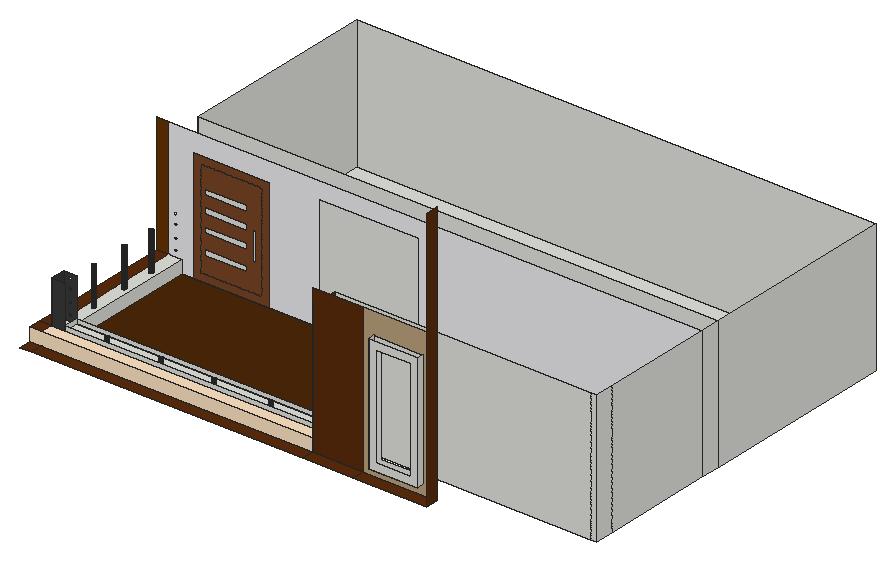
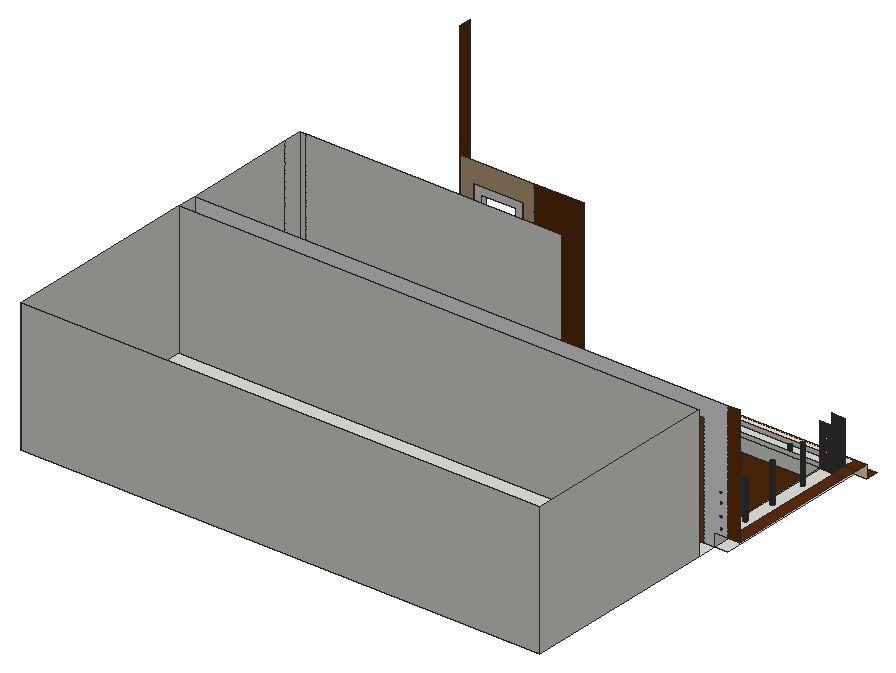
# SketchUp Ruby script. Lengths in inches.
U = 1.inch
M = Sketchup.active_model
def pt(a) = Geom::Point3d.new(a.map { |v| v * U })
def face(e, loops, mat)
  f = e.add_face(loops[0].map { |a| pt(a) })
  loops[1..].each { |l| e.add_face(l.map { |a| pt(a) }).erase! }
  f.material = f.back_material = mat if mat
  f
end
# faces: each face lists its corners as indices into pts; further lists are holes
def faces(e, pts, list, mat = nil) = list.each { |f| face(e, (f[0].is_a?(Array) ? f : [f]).map { |l| l.map { |i| pts[i] } }, mat) }
# xy, xz, yz: faces in a plane at the given z, y or x. An outline is a flat list of corners, or four numbers for a rectangle; further outlines are holes
def ring(l) = l.size == 4 ? [[l[0], l[1]], [l[2], l[1]], [l[2], l[3]], [l[0], l[3]]] : l.each_slice(2).to_a
def flat(e, list, mat, &to3) = list.each { |f| face(e, (f[0].is_a?(Array) ? f : [f]).map { |l| ring(l).map { |u, v| to3.(u, v) } }, mat) }
def xy(e, z, list, mat = nil) = flat(e, list, mat) { |x, y| [x, y, z] }
def xz(e, y, list, mat = nil) = flat(e, list, mat) { |x, z| [x, y, z] }
def yz(e, x, list, mat = nil) = flat(e, list, mat) { |y, z| [x, y, z] }
def lines(e, pts, list) = list.each { |a, b| e.add_line(pt(pts[a]), pt(pts[b])) }
# prism: a flat outline (further loops are holes) pulled along v
def prism(e, loops, v, mat = nil)
  f = face(e, loops, mat); d = Geom::Vector3d.new(v.map { |x| x * U })
  f.pushpull(f.normal.samedirection?(d) ? d.length : -d.length)
end
def box(e, o, s, mat = nil) = prism(e, [[o, [o[0] + s[0], o[1], o[2]], [o[0] + s[0], o[1] + s[1], o[2]], [o[0], o[1] + s[1], o[2]]]], [0, 0, s[2]], mat)
def at(x, y, z, deg = 0) = Geom::Transformation.translation(pt([x, y, z])) * Geom::Transformation.rotation(ORIGIN, Z_AXIS, deg.degrees)
def axes(o, x, y, z) = Geom::Transformation.new([*x, 0, *y, 0, *z, 0, *pt(o).to_a, 1])
def part(name) = M.definitions.add(name)
# library, detail: a bought-in or finely detailed component or shape, given as its bounding box
def library(name, o, s) = part(name).tap { |d| box(d.entities, o, s) }
def detail(e, o, s) = box(e.add_group.entities, o, s)
def put(e, d, t, mat = nil) = e.add_instance(d, t).tap { |i| i.material = mat if mat }
def group(e, t, mat = nil) = e.add_group.tap { |g| g.transformation = t; g.material = mat if mat }.entities
root = M.entities
M.materials.add("[0012_Bisque]").color = [255, 228, 196]
M.materials.add("[0035_Tan]").color = [188, 161, 125]
M.materials.add("[0043_SaddleBrown]").color = [91, 44, 12]
M.materials.add("[Blinds Vertical Pattern]").color = [237, 237, 239]
M.materials.add("[Color C08]").color = [102, 51, 0]
M.materials.add("[Color M07]").color = [58, 58, 58]
M.materials.add("[Leather Red Brown]").color = [76, 40, 8]
M.materials.add("[Wood Veneer 01]").color = [120, 70, 37]
xy(root,141.625,[[73.92,393.34,73.92,538.2,85.98,538.2,85.98,418.04,320.99,418.04,320.99,393.34],[85.98,538.2,560.26,556.28],[85.98,556.28,560.26,737.09]])
xy(root,141.625,[[63.07,382.09,73.92,393.34],[73.92,382.09,320.99,393.34],[320.99,382.09,366.56,393.34],[366.56,382.09,434.25,393.34]],"[0043_SaddleBrown]")
xy(root,141.625,[[85.98,418.04,560.26,538.2]],"[Leather Red Brown]")
xy(root,150.96,[[376.94,386.84,421.82,393.34]])
xy(root,153.1875,[[73.92,404.47,85.98,418.04],[[85.98,404.47,320.99,418.04],[216.94,409.26,217.34,409.31,217.71,409.45,218.03,409.67,218.28,409.95,218.43,410.28,218.48,410.64,218.43,410.99,218.28,411.33,218.03,411.61,217.71,411.83,217.34,411.97,216.94,412.01,216.54,411.97,216.17,411.83,215.85,411.61,215.61,411.33,215.46,410.99,215.4,410.64,215.46,410.28,215.61,409.95,215.85,409.67,216.17,409.45,216.54,409.31],[268.74,409.26,269.14,409.31,269.51,409.45,269.83,409.67,270.08,409.95,270.23,410.28,270.28,410.64,270.23,410.99,270.08,411.33,269.83,411.61,269.51,411.83,269.14,411.97,268.74,412.01,268.34,411.97,267.97,411.83,267.65,411.61,267.41,411.33,267.26,410.99,267.2,410.64,267.26,410.28,267.41,409.95,267.65,409.67,267.97,409.45,268.34,409.31],[168.5,409.26,168.9,409.31,169.27,409.45,169.59,409.67,169.84,409.95,169.99,410.28,170.04,410.64,169.99,410.99,169.84,411.33,169.59,411.61,169.27,411.83,168.9,411.97,168.5,412.01,168.1,411.97,167.73,411.83,167.41,411.61,167.17,411.33,167.02,410.99,166.96,410.64,167.02,410.28,167.17,409.95,167.41,409.67,167.73,409.45,168.1,409.31],[119.01,409.26,119.41,409.31,119.78,409.45,120.1,409.67,120.35,409.95,120.5,410.28,120.55,410.64,120.5,410.99,120.35,411.33,120.1,411.61,119.78,411.83,119.41,411.97,119.01,412.01,118.61,411.97,118.24,411.83,117.92,411.61,117.68,411.33,117.53,410.99,117.47,410.64,117.53,410.28,117.68,409.95,117.92,409.67,118.24,409.45,118.61,409.31]],[119.01,409.26,118.61,409.31,118.24,409.45,117.92,409.67,117.68,409.95,117.53,410.28,117.47,410.64,117.53,410.99,117.68,411.33,117.92,411.61,118.24,411.83,118.61,411.97,119.01,412.01,119.41,411.97,119.78,411.83,120.1,411.61,120.35,411.33,120.5,410.99,120.55,410.64,120.5,410.28,120.35,409.95,120.1,409.67,119.78,409.45,119.41,409.31],[168.5,409.26,168.1,409.31,167.73,409.45,167.41,409.67,167.17,409.95,167.02,410.28,166.96,410.64,167.02,410.99,167.17,411.33,167.41,411.61,167.73,411.83,168.1,411.97,168.5,412.01,168.9,411.97,169.27,411.83,169.59,411.61,169.84,411.33,169.99,410.99,170.04,410.64,169.99,410.28,169.84,409.95,169.59,409.67,169.27,409.45,168.9,409.31],[216.94,409.26,216.54,409.31,216.17,409.45,215.85,409.67,215.61,409.95,215.46,410.28,215.4,410.64,215.46,410.99,215.61,411.33,215.85,411.61,216.17,411.83,216.54,411.97,216.94,412.01,217.34,411.97,217.71,411.83,218.03,411.61,218.28,411.33,218.43,410.99,218.48,410.64,218.43,410.28,218.28,409.95,218.03,409.67,217.71,409.45,217.34,409.31],
  [268.74,409.26,268.34,409.31,267.97,409.45,267.65,409.67,267.41,409.95,267.26,410.28,267.2,410.64,267.26,410.99,267.41,411.33,267.65,411.61,267.97,411.83,268.34,411.97,268.74,412.01,269.14,411.97,269.51,411.83,269.83,411.61,270.08,411.33,270.23,410.99,270.28,410.64,270.23,410.28,270.08,409.95,269.83,409.67,269.51,409.45,269.14,409.31],[[73.92,418.04,85.98,538.2],[80.02,443.08,79.56,443.13,79.14,443.29,78.78,443.54,78.5,443.86,78.33,444.24,78.27,444.64,78.33,445.05,78.5,445.42,78.78,445.75,79.14,445.99,79.56,446.15,80.02,446.2,80.47,446.15,80.89,445.99,81.25,445.75,81.53,445.42,81.71,445.05,81.77,444.64,81.71,444.24,81.53,443.86,81.25,443.54,80.89,443.29,80.47,443.13],[80.02,477.83,79.56,477.88,79.14,478.04,78.78,478.29,78.5,478.61,78.33,478.99,78.27,479.39,78.33,479.8,78.5,480.17,78.78,480.5,79.14,480.74,79.56,480.9,80.02,480.95,80.47,480.9,80.89,480.74,81.25,480.5,81.53,480.17,81.71,479.8,81.77,479.39,81.71,478.99,81.53,478.61,81.25,478.29,80.89,478.04,80.47,477.88],[80.02,508.58,79.56,508.63,79.14,508.79,78.78,509.04,78.5,509.36,78.33,509.74,78.27,510.14,78.33,510.55,78.5,510.92,78.78,511.25,79.14,511.49,79.56,511.65,80.02,511.7,80.47,511.65,80.89,511.49,81.25,511.25,81.53,510.92,81.71,510.55,81.77,510.14,81.71,509.74,81.53,509.36,81.25,509.04,80.89,508.79,80.47,508.63]],[80.02,443.08,79.56,443.13,79.14,443.29,78.78,443.54,78.5,443.86,78.33,444.24,78.27,444.64,78.33,445.05,78.5,445.42,78.78,445.75,79.14,445.99,79.56,446.15,80.02,446.2,80.47,446.15,80.89,445.99,81.25,445.75,81.53,445.42,81.71,445.05,81.77,444.64,81.71,444.24,81.53,443.86,81.25,443.54,80.89,443.29,80.47,443.13],[80.02,477.83,79.56,477.88,79.14,478.04,78.78,478.29,78.5,478.61,78.33,478.99,78.27,479.39,78.33,479.8,78.5,480.17,78.78,480.5,79.14,480.74,79.56,480.9,80.02,480.95,80.47,480.9,80.89,480.74,81.25,480.5,81.53,480.17,81.71,479.8,81.77,479.39,81.71,478.99,81.53,478.61,81.25,478.29,80.89,478.04,80.47,477.88],[80.02,508.58,79.56,508.63,79.14,508.79,78.78,509.04,78.5,509.36,78.33,509.74,78.27,510.14,78.33,510.55,78.5,510.92,78.78,511.25,79.14,511.49,79.56,511.65,80.02,511.7,80.47,511.65,80.89,511.49,81.25,511.25,81.53,510.92,81.71,510.55,81.77,510.14,81.71,509.74,81.53,509.36,81.25,509.04,80.89,508.79,80.47,508.63]])
xy(root,153.1875,[[73.92,393.34,320.99,404.47]],"[0012_Bisque]")
xy(root,153.1875,[[63.07,393.34,73.92,404.47],[63.07,404.47,73.92,418.04],[63.07,418.04,73.92,538.2]],"[0043_SaddleBrown]")
xz(root,386.84,[[[376.94,150.96,421.82,257.08],[383.5,157.51,415.27,250.53]]])
xz(root,393.34,[[[376.94,150.96,421.82,257.08],[383.5,157.51,415.27,250.53]]])
xz(root,393.34,[[63.07,141.625,320.99,153.1875]],"[0012_Bisque]")
xz(root,393.34,[[[366.56,141.625,434.25,276.4375],[376.94,150.96,421.82,257.08]]],"[0035_Tan]")
xz(root,393.34,[[320.99,141.625,366.56,276.4375]],"[0043_SaddleBrown]")
xz(root,404.47,[[85.98,153.1875,320.99,157.625]])
xz(root,404.47,[[73.92,153.1875,85.98,192.1875]],"[Color M07]")
xz(root,418.04,[[85.98,141.625,320.99,153.1875],[320.99,141.625,554.62,261.625],[554.62,141.625,560.26,261.625],[85.98,153.1875,320.99,157.625]])
xz(root,418.04,[[[73.92,153.1875,85.98,192.1875],[79.95,186.93,80.37,186.98,80.75,187.12,81.09,187.35,81.34,187.65,81.5,187.99,81.56,188.37,81.5,188.74,81.34,189.08,81.09,189.38,80.75,189.61,80.37,189.75,79.95,189.8,79.53,189.75,79.14,189.61,78.8125,189.38,78.55,189.08,78.39,188.74,78.34,188.37,78.39,187.99,78.55,187.65,78.8125,187.35,79.14,187.12,79.53,186.98],[79.95,178.37,80.37,178.41,80.75,178.56,81.09,178.79,81.34,179.08,81.5,179.43,81.56,179.8,81.5,180.17,81.34,180.52,81.09,180.82,80.75,181.05,80.37,181.19,79.95,181.24,79.53,181.19,79.14,181.05,78.8125,180.82,78.55,180.52,78.39,180.17,78.34,179.8,78.39,179.43,78.55,179.08,78.8125,178.79,79.14,178.56,79.53,178.41],[79.95,166.99,80.37,167.04,80.75,167.18,81.09,167.41,81.34,167.71,81.5,168.06,81.56,168.43,81.5,168.8,81.34,169.15,81.09,169.44,80.75,169.67,80.37,169.82,79.95,169.87,79.53,169.82,79.14,169.67,78.8125,169.44,78.55,169.15,78.39,168.8,78.34,168.43,78.39,168.06,78.55,167.71,78.8125,167.41,79.14,167.18,79.53,167.04],[79.95,156.99,80.37,157.04,80.75,157.18,81.09,157.41,81.34,157.71,81.5,158.06,81.56,158.43,81.5,158.8,81.34,159.15,81.09,159.44,80.75,159.67,80.37,159.82,79.95,159.87,79.53,159.82,79.14,159.67,78.8125,159.44,78.55,159.15,78.39,158.8,78.34,158.43,78.39,158.06,78.55,157.71,78.8125,157.41,79.14,157.18,79.53,157.04]]],"[Color M07]")
xz(root,538.2,[[[85.98,141.625,95.27,141.625,95.27,244.07,166.18,244.07,166.18,141.625,560.26,141.625,560.26,261.625,73.92,261.625,73.92,153.1875,85.98,153.1875],[211.03,165.38,301.61,246.26],[79.95,156.99,79.53,157.04,79.14,157.18,78.8125,157.41,78.55,157.71,78.39,158.06,78.34,158.43,78.39,158.8,78.55,159.15,78.8125,159.44,79.14,159.67,79.53,159.82,79.95,159.87,80.37,159.82,80.75,159.67,81.09,159.44,81.34,159.15,81.5,158.8,81.56,158.43,81.5,158.06,81.34,157.71,81.09,157.41,80.75,157.18,80.37,157.04],[79.95,186.93,79.53,186.98,79.14,187.12,78.8125,187.35,78.55,187.65,78.39,187.99,78.34,188.37,78.39,188.74,78.55,189.08,78.8125,189.38,79.14,189.61,79.53,189.75,79.95,189.8,80.37,189.75,80.75,189.61,81.09,189.38,81.34,189.08,81.5,188.74,81.56,188.37,81.5,187.99,81.34,187.65,81.09,187.35,80.75,187.12,80.37,186.98],[79.95,166.99,79.53,167.04,79.14,167.18,78.8125,167.41,78.55,167.71,78.39,168.06,78.34,168.43,78.39,168.8,78.55,169.15,78.8125,169.44,79.14,169.67,79.53,169.82,79.95,169.87,80.37,169.82,80.75,169.67,81.09,169.44,81.34,169.15,81.5,168.8,81.56,168.43,81.5,168.06,81.34,167.71,81.09,167.41,80.75,167.18,80.37,167.04],[79.95,178.37,79.53,178.41,79.14,178.56,78.8125,178.79,78.55,179.08,78.39,179.43,78.34,179.8,78.39,180.17,78.55,180.52,78.8125,180.82,79.14,181.05,79.53,181.19,79.95,181.24,80.37,181.19,80.75,181.05,81.09,180.82,81.34,180.52,81.5,180.17,81.56,179.8,81.5,179.43,81.34,179.08,81.09,178.79,80.75,178.56,80.37,178.41]]],"[Blinds Vertical Pattern]")
xz(root,538.2,[[63.07,153.1875,73.92,261.625]],"[Color C08]")
xz(root,538.2,[[[95.27,141.625,166.18,244.07],[102.77,148.32,158.68,237.37]],[[102.77,148.32,158.68,237.37],[106.17,212.92,145.09,218.23],[106.17,197.6,145.09,202.92],[106.17,181.73,145.09,187.04],[106.17,163.54,145.09,168.85],[149.97,173.81,153.54,199.88]]],"[Wood Veneer 01]")
xz(root,556.28,[[85.98,141.625,560.26,261.625]])
xz(root,737.09,[[85.98,141.625,560.26,261.625]])
yz(root,73.92,[[404.47,153.1875,418.04,192.1875]],"[Color M07]")
yz(root,85.98,[[418.04,141.625,538.2,153.1875],[556.28,141.625,737.09,261.625],[404.47,153.1875,404.47,157.625,409.74,157.625,410.08,157.37,410.53,157.18,411.02,157.12,411.5,157.18,411.95,157.37,412.29,157.625,418.04,157.625,418.04,153.1875]])
yz(root,320.99,[[393.34,141.625,418.04,153.1875],[404.47,153.1875,404.47,157.625,409.74,157.625,410.08,157.37,410.53,157.18,411.02,157.12,411.5,157.18,411.95,157.37,412.29,157.625,418.04,157.625,418.04,153.1875]])
yz(root,320.99,[[[393.34,153.1875,393.34,261.625,418.04,261.625,418.04,157.625,412.29,157.625,412.34,157.67,412.64,158.06,412.83,158.51,412.89,158.99,412.83,159.48,412.64,159.93,412.34,160.32,411.95,160.62,411.5,160.8,411.02,160.87,410.53,160.8,410.08,160.62,409.69,160.32,409.39,159.93,409.2,159.48,409.14,158.99,409.2,158.51,409.39,158.06,409.69,157.67,409.74,157.625,404.47,157.625,404.47,153.1875],[411.02,166.87,411.5,166.93,411.95,167.12,412.34,167.42,412.64,167.81,412.83,168.26,412.89,168.74,412.83,169.23,412.64,169.68,412.34,170.07,411.95,170.37,411.5,170.55,411.02,170.62,410.53,170.55,410.08,170.37,409.69,170.07,409.39,169.68,409.2,169.23,409.14,168.74,409.2,168.26,409.39,167.81,409.69,167.42,410.08,167.12,410.53,166.93],[411.02,177.37,411.5,177.43,411.95,177.62,412.34,177.92,412.64,178.31,412.83,178.76,412.89,179.24,412.83,179.73,412.64,180.18,412.34,180.57,411.95,180.87,411.5,181.05,411.02,181.12,410.53,181.05,410.08,180.87,409.69,180.57,409.39,180.18,409.2,179.73,409.14,179.24,409.2,178.76,409.39,178.31,409.69,177.92,410.08,177.62,410.53,177.43],[411.02,186.49,411.5,186.56,411.95,186.74,412.34,187.04,412.64,187.43,412.83,187.88,412.89,188.37,412.83,188.85,412.64,189.31,412.34,189.69,411.95,189.99,411.5,190.18,411.02,190.24,410.53,190.18,410.08,189.99,409.69,189.69,409.39,189.31,409.2,188.85,409.14,188.37,409.2,187.88,409.39,187.43,409.69,187.04,410.08,186.74,410.53,186.56]]],"[0043_SaddleBrown]")
yz(root,376.94,[[386.84,150.96,393.34,257.08]])
yz(root,421.82,[[386.84,150.96,393.34,257.08]])
yz(root,434.25,[[382.09,141.625,393.34,381.625]],"[0043_SaddleBrown]")
yz(root,560.26,[[418.04,141.625,434.85,261.625],[434.85,141.625,538.2,261.625],[538.2,141.625,556.28,261.625],[556.28,141.625,737.09,261.625]])
p = [[118.24,409.45,153.1875],[118.61,409.31,153.1875],[118.61,409.31,157.625],[118.24,409.45,157.625],[119.01,409.26,153.1875],[119.01,409.26,157.625],
  [119.41,409.31,153.1875],[119.41,409.31,157.625],[119.78,409.45,153.1875],[119.78,409.45,157.625],[167.73,409.45,153.1875],[168.1,409.31,153.1875],
  [168.1,409.31,157.625],[167.73,409.45,157.625],[168.5,409.26,153.1875],[168.5,409.26,157.625],[168.9,409.31,153.1875],[168.9,409.31,157.625],
  [169.27,409.45,153.1875],[169.27,409.45,157.625],[216.17,409.45,153.1875],[216.54,409.31,153.1875],[216.54,409.31,157.625],[216.17,409.45,157.625],
  [216.94,409.26,153.1875],[216.94,409.26,157.625],[217.34,409.31,153.1875],[217.34,409.31,157.625],[217.71,409.45,153.1875],[217.71,409.45,157.625],
  [267.97,409.45,153.1875],[268.34,409.31,153.1875],[268.34,409.31,157.625],[267.97,409.45,157.625],[268.74,409.26,153.1875],[268.74,409.26,157.625],
  [269.14,409.31,153.1875],[269.14,409.31,157.625],[269.51,409.45,153.1875],[269.51,409.45,157.625],[117.92,409.67,153.1875],[117.92,409.67,157.625],
  [120.1,409.67,153.1875],[120.1,409.67,157.625],[167.41,409.67,153.1875],[167.41,409.67,157.625],[169.59,409.67,153.1875],[169.59,409.67,157.625],
  [215.85,409.67,153.1875],[215.85,409.67,157.625],[218.03,409.67,153.1875],[218.03,409.67,157.625],[267.65,409.67,153.1875],[267.65,409.67,157.625],
  [269.83,409.67,153.1875],[269.83,409.67,157.625],[117.68,409.95,153.1875],[117.68,409.95,157.625],[120.35,409.95,153.1875],[120.35,409.95,157.625],
  [167.17,409.95,153.1875],[167.17,409.95,157.625],[169.84,409.95,153.1875],[169.84,409.95,157.625],[215.61,409.95,153.1875],[215.61,409.95,157.625],
  [218.28,409.95,153.1875],[218.28,409.95,157.625],[267.41,409.95,153.1875],[267.41,409.95,157.625],[270.08,409.95,153.1875],[270.08,409.95,157.625],
  [117.53,410.28,153.1875],[117.53,410.28,157.625],[120.5,410.28,153.1875],[120.5,410.28,157.625],[167.02,410.28,153.1875],[167.02,410.28,157.625],
  [169.99,410.28,153.1875],[169.99,410.28,157.625],[215.46,410.28,153.1875],[215.46,410.28,157.625],[218.43,410.28,153.1875],[218.43,410.28,157.625],
  [267.26,410.28,153.1875],[267.26,410.28,157.625],[270.23,410.28,153.1875],[270.23,410.28,157.625],[117.47,410.64,153.1875],[117.47,410.64,157.625],
  [120.55,410.64,153.1875],[120.55,410.64,157.625],[166.96,410.64,153.1875],[166.96,410.64,157.625],[170.04,410.64,153.1875],[170.04,410.64,157.625],
  [215.4,410.64,153.1875],[215.4,410.64,157.625],[218.48,410.64,153.1875],[218.48,410.64,157.625],[267.2,410.64,153.1875],[267.2,410.64,157.625],
  [270.28,410.64,153.1875],[270.28,410.64,157.625],[117.53,410.99,153.1875],[117.53,410.99,157.625],[120.5,410.99,153.1875],[120.5,410.99,157.625],
  [167.02,410.99,153.1875],[167.02,410.99,157.625],[169.99,410.99,153.1875],[169.99,410.99,157.625],[215.46,410.99,153.1875],[215.46,410.99,157.625],
  [218.43,410.99,153.1875],[218.43,410.99,157.625],[267.26,410.99,153.1875],[267.26,410.99,157.625],[270.23,410.99,153.1875],[270.23,410.99,157.625],
  [117.68,411.33,153.1875],[117.68,411.33,157.625],[120.35,411.33,153.1875],[120.35,411.33,157.625],[167.17,411.33,153.1875],[167.17,411.33,157.625],
  [169.84,411.33,153.1875],[169.84,411.33,157.625],[215.61,411.33,153.1875],[215.61,411.33,157.625],[218.28,411.33,153.1875],[218.28,411.33,157.625],
  [267.41,411.33,153.1875],[267.41,411.33,157.625],[270.08,411.33,153.1875],[270.08,411.33,157.625],[117.92,411.61,153.1875],[117.92,411.61,157.625],
  [120.1,411.61,153.1875],[120.1,411.61,157.625],[167.41,411.61,153.1875],[167.41,411.61,157.625],[169.59,411.61,153.1875],[169.59,411.61,157.625],
  [215.85,411.61,153.1875],[215.85,411.61,157.625],[218.03,411.61,153.1875],[218.03,411.61,157.625],[267.65,411.61,153.1875],[267.65,411.61,157.625],
  [269.83,411.61,153.1875],[269.83,411.61,157.625],[118.24,411.83,153.1875],[118.24,411.83,157.625],[119.78,411.83,153.1875],[119.78,411.83,157.625],
  [167.73,411.83,153.1875],[167.73,411.83,157.625],[169.27,411.83,153.1875],[169.27,411.83,157.625],[216.17,411.83,153.1875],[216.17,411.83,157.625],
  [217.71,411.83,153.1875],[217.71,411.83,157.625],[267.97,411.83,153.1875],[267.97,411.83,157.625],[269.51,411.83,153.1875],[269.51,411.83,157.625],
  [118.61,411.97,153.1875],[118.61,411.97,157.625],[119.41,411.97,153.1875],[119.41,411.97,157.625],[168.1,411.97,153.1875],[168.1,411.97,157.625],
  [168.9,411.97,153.1875],[168.9,411.97,157.625],[216.54,411.97,153.1875],[216.54,411.97,157.625],[217.34,411.97,153.1875],[217.34,411.97,157.625],
  [268.34,411.97,153.1875],[268.34,411.97,157.625],[269.14,411.97,153.1875],[269.14,411.97,157.625],[119.01,412.01,153.1875],[119.01,412.01,157.625],
  [168.5,412.01,153.1875],[168.5,412.01,157.625],[216.94,412.01,153.1875],[216.94,412.01,157.625],[268.74,412.01,153.1875],[268.74,412.01,157.625],
  [79.14,443.29,153.1875],[79.56,443.13,153.1875],[79.56,443.13,187.8125],[79.14,443.29,187.8125],[80.02,443.08,153.1875],[80.02,443.08,187.8125],
  [80.47,443.13,153.1875],[80.47,443.13,187.8125],[80.89,443.29,153.1875],[80.89,443.29,187.8125],[78.78,443.54,153.1875],[78.78,443.54,187.8125],
  [81.25,443.54,153.1875],[81.25,443.54,187.8125],[78.5,443.86,153.1875],[78.5,443.86,187.8125],[81.53,443.86,153.1875],[81.53,443.86,187.8125],
  [78.33,444.24,153.1875],[78.33,444.24,187.8125],[81.71,444.24,153.1875],[81.71,444.24,187.8125],[78.27,444.64,153.1875],[78.27,444.64,187.8125],
  [81.77,444.64,153.1875],[81.77,444.64,187.8125],[78.33,445.05,153.1875],[78.33,445.05,187.8125],[81.71,445.05,153.1875],[81.71,445.05,187.8125],
  [78.5,445.42,153.1875],[78.5,445.42,187.8125],[81.53,445.42,153.1875],[81.53,445.42,187.8125],[78.78,445.75,153.1875],[78.78,445.75,187.8125],
  [81.25,445.75,153.1875],[81.25,445.75,187.8125],[79.14,445.99,153.1875],[79.14,445.99,187.8125],[80.89,445.99,153.1875],[80.89,445.99,187.8125],
  [79.56,446.15,153.1875],[79.56,446.15,187.8125],[80.47,446.15,153.1875],[80.47,446.15,187.8125],[80.02,446.2,153.1875],[80.02,446.2,187.8125],
  [79.56,477.88,153.1875],[80.02,477.83,153.1875],[80.02,477.83,188.1875],[79.56,477.88,188.1875],[80.47,477.88,153.1875],[80.47,477.88,188.1875],
  [79.14,478.04,153.1875],[79.14,478.04,188.1875],[80.89,478.04,153.1875],[80.89,478.04,188.1875],[78.78,478.29,153.1875],[78.78,478.29,188.1875],
  [81.25,478.29,153.1875],[81.25,478.29,188.1875],[78.5,478.61,153.1875],[78.5,478.61,188.1875],[81.53,478.61,153.1875],[81.53,478.61,188.1875],
  [78.33,478.99,153.1875],[78.33,478.99,188.1875],[81.71,478.99,153.1875],[81.71,478.99,188.1875],[78.27,479.39,153.1875],[78.27,479.39,188.1875],
  [81.77,479.39,153.1875],[81.77,479.39,188.1875],[78.33,479.8,153.1875],[78.33,479.8,188.1875],[81.71,479.8,153.1875],[81.71,479.8,188.1875],
  [78.5,480.17,153.1875],[78.5,480.17,188.1875],[81.53,480.17,153.1875],[81.53,480.17,188.1875],[78.78,480.5,153.1875],[78.78,480.5,188.1875],
  [81.25,480.5,153.1875],[81.25,480.5,188.1875],[79.14,480.74,153.1875],[79.14,480.74,188.1875],[80.89,480.74,153.1875],[80.89,480.74,188.1875],
  [79.56,480.9,153.1875],[79.56,480.9,188.1875],[80.47,480.9,153.1875],[80.47,480.9,188.1875],[80.02,480.95,153.1875],[80.02,480.95,188.1875],
  [79.14,508.79,153.1875],[79.56,508.63,153.1875],[79.56,508.63,187.6875],[79.14,508.79,187.6875],[80.02,508.58,153.1875],[80.02,508.58,187.6875],
  [80.47,508.63,153.1875],[80.47,508.63,187.6875],[80.89,508.79,153.1875],[80.89,508.79,187.6875],[78.78,509.04,153.1875],[78.78,509.04,187.6875],
  [81.25,509.04,153.1875],[81.25,509.04,187.6875],[78.5,509.36,153.1875],[78.5,509.36,187.6875],[81.53,509.36,153.1875],[81.53,509.36,187.6875],
  [78.33,509.74,153.1875],[78.33,509.74,187.6875],[81.71,509.74,153.1875],[81.71,509.74,187.6875],[78.27,510.14,153.1875],[78.27,510.14,187.6875],
  [81.77,510.14,153.1875],[81.77,510.14,187.6875],[78.33,510.55,153.1875],[78.33,510.55,187.6875],[81.71,510.55,153.1875],[81.71,510.55,187.6875],
  [78.5,510.92,153.1875],[78.5,510.92,187.6875],[81.53,510.92,153.1875],[81.53,510.92,187.6875],[78.78,511.25,153.1875],[78.78,511.25,187.6875],
  [81.25,511.25,153.1875],[81.25,511.25,187.6875],[79.14,511.49,153.1875],[79.14,511.49,187.6875],[80.89,511.49,153.1875],[80.89,511.49,187.6875],
  [79.56,511.65,153.1875],[79.56,511.65,187.6875],[80.47,511.65,153.1875],[80.47,511.65,187.6875],[80.02,511.7,153.1875],[80.02,511.7,187.6875]]
faces(root,p,[[0,1,2,3],[1,4,5,2],[4,6,7,5],[6,8,9,7],[10,11,12,13],[11,14,15,12],[14,16,17,15],[16,18,19,17],
  [20,21,22,23],[21,24,25,22],[24,26,27,25],[26,28,29,27],[30,31,32,33],[31,34,35,32],[34,36,37,35],[36,38,39,37],
  [40,0,3,41],[8,42,43,9],[44,10,13,45],[18,46,47,19],[48,20,23,49],[28,50,51,29],[52,30,33,53],[38,54,55,39],
  [56,40,41,57],[42,58,59,43],[60,44,45,61],[46,62,63,47],[64,48,49,65],[50,66,67,51],[68,52,53,69],[54,70,71,55],
  [72,56,57,73],[58,74,75,59],[76,60,61,77],[62,78,79,63],[80,64,65,81],[66,82,83,67],[84,68,69,85],[70,86,87,71],
  [88,72,73,89],[74,90,91,75],[92,76,77,93],[78,94,95,79],[96,80,81,97],[82,98,99,83],[100,84,85,101],[86,102,103,87],
  [104,88,89,105],[90,106,107,91],[108,92,93,109],[94,110,111,95],[112,96,97,113],[98,114,115,99],[116,100,101,117],[102,118,119,103],
  [120,104,105,121],[106,122,123,107],[124,108,109,125],[110,126,127,111],[128,112,113,129],[114,130,131,115],[132,116,117,133],[118,134,135,119],
  [136,120,121,137],[122,138,139,123],[140,124,125,141],[126,142,143,127],[144,128,129,145],[130,146,147,131],[148,132,133,149],[134,150,151,135],
  [152,136,137,153],[138,154,155,139],[156,140,141,157],[142,158,159,143],[160,144,145,161],[146,162,163,147],[164,148,149,165],[150,166,167,151],
  [168,152,153,169],[154,170,171,155],[172,156,157,173],[158,174,175,159],[176,160,161,177],[162,178,179,163],[180,164,165,181],[166,182,183,167],
  [184,168,169,185],[170,184,185,171],[186,172,173,187],[174,186,187,175],[188,176,177,189],[178,188,189,179],[190,180,181,191],[182,190,191,183]])
faces(root,p,[[192,193,194,195],[193,196,197,194],[196,198,199,197],[198,200,201,199],[202,192,195,203],[200,204,205,201],[206,202,203,207],[204,208,209,205],
  [210,206,207,211],[208,212,213,209],[214,210,211,215],[212,216,217,213],[218,214,215,219],[216,220,221,217],[222,218,219,223],[220,224,225,221],
  [226,222,223,227],[224,228,229,225],[230,226,227,231],[228,232,233,229],[234,230,231,235],[232,236,237,233],[238,234,235,239],[236,238,239,237],
  [240,241,242,243],[241,244,245,242],[246,240,243,247],[244,248,249,245],[250,246,247,251],[248,252,253,249],[254,250,251,255],[252,256,257,253],
  [258,254,255,259],[256,260,261,257],[262,258,259,263],[260,264,265,261],[266,262,263,267],[264,268,269,265],[270,266,267,271],[268,272,273,269],
  [274,270,271,275],[272,276,277,273],[278,274,275,279],[276,280,281,277],[282,278,279,283],[280,284,285,281],[286,282,283,287],[284,286,287,285],
  [288,289,290,291],[289,292,293,290],[292,294,295,293],[294,296,297,295],[298,288,291,299],[296,300,301,297],[302,298,299,303],[300,304,305,301],
  [306,302,303,307],[304,308,309,305],[310,306,307,311],[308,312,313,309],[314,310,311,315],[312,316,317,313],[318,314,315,319],[316,320,321,317],
  [322,318,319,323],[320,324,325,321],[326,322,323,327],[324,328,329,325],[330,326,327,331],[328,332,333,329],[334,330,331,335],[332,334,335,333]],"[Color M07]")
